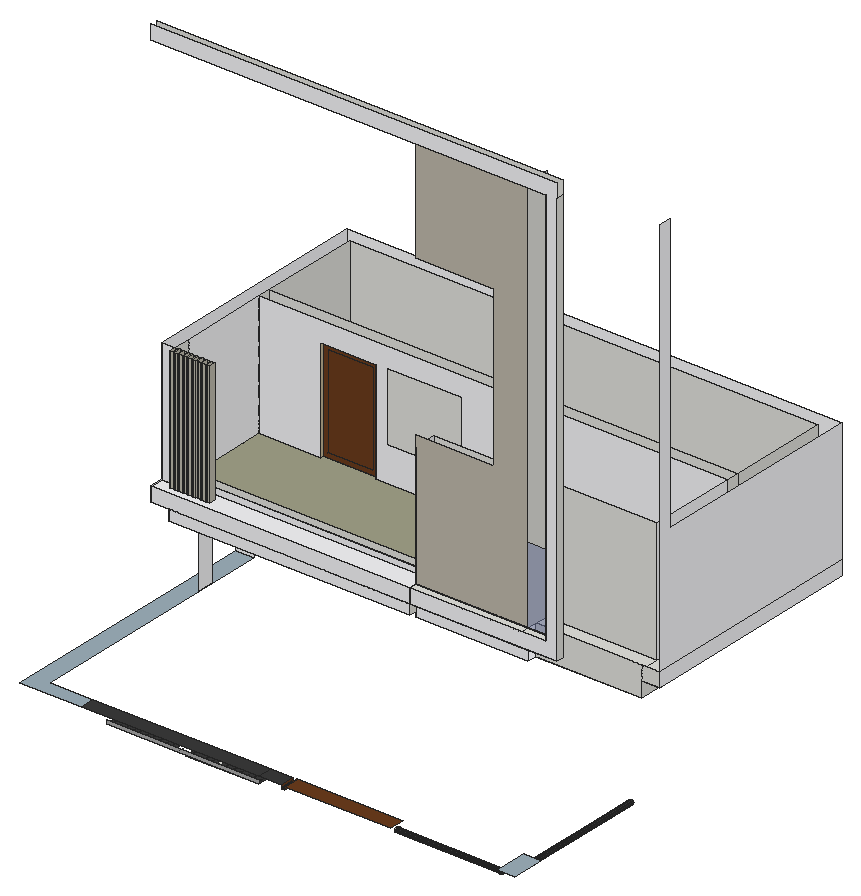
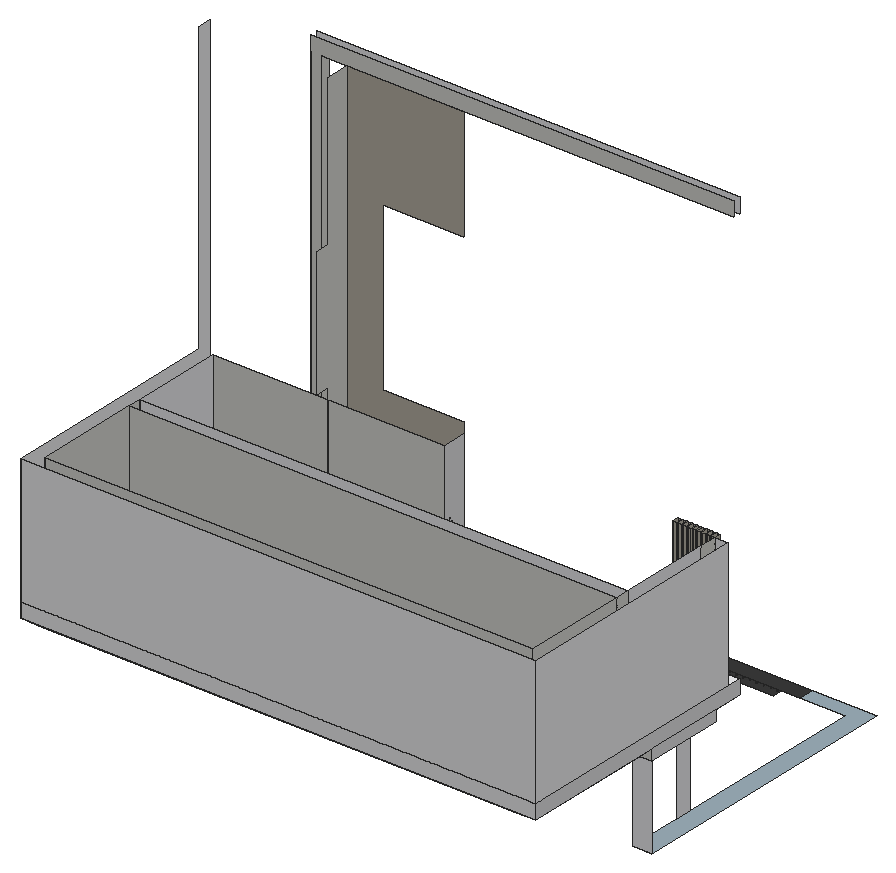
# SketchUp Ruby script. Lengths in inches.
U = 1.inch
M = Sketchup.active_model
def pt(a) = Geom::Point3d.new(a.map { |v| v * U })
def face(e, loops, mat)
  f = e.add_face(loops[0].map { |a| pt(a) })
  loops[1..].each { |l| e.add_face(l.map { |a| pt(a) }).erase! }
  f.material = f.back_material = mat if mat
  f
end
# faces: each face lists its corners as indices into pts; further lists are holes
def faces(e, pts, list, mat = nil) = list.each { |f| face(e, (f[0].is_a?(Array) ? f : [f]).map { |l| l.map { |i| pts[i] } }, mat) }
# xy, xz, yz: faces in a plane at the given z, y or x. An outline is a flat list of corners, or four numbers for a rectangle; further outlines are holes
def ring(l) = l.size == 4 ? [[l[0], l[1]], [l[2], l[1]], [l[2], l[3]], [l[0], l[3]]] : l.each_slice(2).to_a
def flat(e, list, mat, &to3) = list.each { |f| face(e, (f[0].is_a?(Array) ? f : [f]).map { |l| ring(l).map { |u, v| to3.(u, v) } }, mat) }
def xy(e, z, list, mat = nil) = flat(e, list, mat) { |x, y| [x, y, z] }
def xz(e, y, list, mat = nil) = flat(e, list, mat) { |x, z| [x, y, z] }
def yz(e, x, list, mat = nil) = flat(e, list, mat) { |y, z| [x, y, z] }
def lines(e, pts, list) = list.each { |a, b| e.add_line(pt(pts[a]), pt(pts[b])) }
# prism: a flat outline (further loops are holes) pulled along v
def prism(e, loops, v, mat = nil)
  f = face(e, loops, mat); d = Geom::Vector3d.new(v.map { |x| x * U })
  f.pushpull(f.normal.samedirection?(d) ? d.length : -d.length)
end
def box(e, o, s, mat = nil) = prism(e, [[o, [o[0] + s[0], o[1], o[2]], [o[0] + s[0], o[1] + s[1], o[2]], [o[0], o[1] + s[1], o[2]]]], [0, 0, s[2]], mat)
def at(x, y, z, deg = 0) = Geom::Transformation.translation(pt([x, y, z])) * Geom::Transformation.rotation(ORIGIN, Z_AXIS, deg.degrees)
def axes(o, x, y, z) = Geom::Transformation.new([*x, 0, *y, 0, *z, 0, *pt(o).to_a, 1])
def part(name) = M.definitions.add(name)
# library, detail: a bought-in or finely detailed component or shape, given as its bounding box
def library(name, o, s) = part(name).tap { |d| box(d.entities, o, s) }
def detail(e, o, s) = box(e.add_group.entities, o, s)
def put(e, d, t, mat = nil) = e.add_instance(d, t).tap { |i| i.material = mat if mat }
def group(e, t, mat = nil) = e.add_group.tap { |g| g.transformation = t; g.material = mat if mat }.entities
root = M.entities
M.materials.add("[Asphalt New]").color = [67, 60, 62]
M.materials.add("[Blinds Vertical Pattern]").color = [245, 245, 247]
M.materials.add("[Blinds Vertical Pattern]2").color = [234, 234, 237]
M.materials.add("[Blinds Vertical Pattern]3").color = [247, 247, 249]
M.materials.add("[Cinder Block]").color = [191, 184, 171]
M.materials.add("[Color M03]").color = [170, 170, 170]
M.materials.add("[Color M07]").color = [58, 58, 58]
M.materials.add("[Fabric Linen]").color = [161, 161, 136]
M.materials.add("[Formica Beige]").color = [211, 187, 149]
M.materials.add("[Formica Graystone]").color = [191, 187, 173]
M.materials.add("[Formica Speckled Grey]").color = [157, 176, 186]
M.materials.add("[Quartz Light Brown]").color = [199, 184, 152]
M.materials.add("[Quartz Light Grey]").color = [251, 251, 252]
M.materials.add("[Translucent Glass Sky Reflection]").color = [126, 138, 183]
M.materials["[Translucent Glass Sky Reflection]"].alpha = 0.52
M.materials.add("[Wood Cherry Original]").color = [107, 60, 29]
xy(root,112.6,[[[163.91,195.25,260.48,216.53],[167.65,202.87,168.24,202.95,168.8,203.18,169.28,203.55,169.65,204.03,169.88,204.58,169.96,205.18,169.88,205.78,169.65,206.34,169.28,206.82,168.8,207.18,168.24,207.42,167.65,207.49,167.05,207.42,166.49,207.18,166.01,206.82,165.64,206.34,165.41,205.78,165.33,205.18,165.41,204.58,165.64,204.03,166.01,203.55,166.49,203.18,167.05,202.95],[176.58,202.87,177.18,202.95,177.74,203.18,178.22,203.55,178.59,204.03,178.82,204.58,178.9,205.18,178.82,205.78,178.59,206.34,178.22,206.82,177.74,207.18,177.18,207.42,176.58,207.49,175.98,207.42,175.43,207.18,174.95,206.82,174.58,206.34,174.35,205.78,174.27,205.18,174.35,204.58,174.58,204.03,174.95,203.55,175.43,203.18,175.98,202.95],[186.9,202.87,187.49,202.95,188.05,203.18,188.53,203.55,188.9,204.03,189.13,204.58,189.21,205.18,189.13,205.78,188.9,206.34,188.53,206.82,188.05,207.18,187.49,207.42,186.9,207.49,186.3,207.42,185.74,207.18,185.26,206.82,184.89,206.34,184.66,205.78,184.58,205.18,184.66,204.58,184.89,204.03,185.26,203.55,185.74,203.18,186.3,202.95],[196.21,202.87,196.81,202.95,197.36,203.18,197.84,203.55,198.21,204.03,198.44,204.58,198.52,205.18,198.44,205.78,198.21,206.34,197.84,206.82,197.36,207.18,196.81,207.42,196.21,207.49,195.61,207.42,195.05,207.18,194.57,206.82,194.21,206.34,193.97,205.78,193.9,205.18,193.97,204.58,194.21,204.03,194.57,203.55,195.05,203.18,195.61,202.95],[205.65,202.87,206.24,202.95,206.8,203.18,207.28,203.55,207.65,204.03,207.88,204.58,207.96,205.18,207.88,205.78,207.65,206.34,207.28,206.82,206.8,207.18,206.24,207.42,205.65,207.49,205.05,207.42,204.49,207.18,204.01,206.82,203.64,206.34,203.41,205.78,203.33,205.18,203.41,204.58,203.64,204.03,204.01,203.55,204.49,203.18,205.05,202.95],[215.27,202.87,215.87,202.95,216.43,203.18,216.91,203.55,217.27,204.03,217.5,204.58,217.58,205.18,217.5,205.78,217.27,206.34,216.91,206.82,216.43,207.18,215.87,207.42,215.27,207.49,214.67,207.42,214.11,207.18,213.64,206.82,213.27,206.34,213.04,205.78,212.96,205.18,213.04,204.58,213.27,204.03,213.64,203.55,214.11,203.18,214.67,202.95],[224.83,202.87,225.43,202.95,225.99,203.18,226.47,203.55,226.84,204.03,227.07,204.58,227.15,205.18,227.07,205.78,226.84,206.34,226.47,206.82,225.99,207.18,225.43,207.42,224.83,207.49,224.23,207.42,223.68,207.18,223.2,206.82,222.83,206.34,222.6,205.78,222.52,205.18,222.6,204.58,222.83,204.03,223.2,203.55,223.68,203.18,224.23,202.95],[234.71,202.87,235.31,202.95,235.86,203.18,236.34,203.55,236.71,204.03,236.94,204.58,237.02,205.18,236.94,205.78,236.71,206.34,236.34,206.82,235.86,207.18,235.31,207.42,234.71,207.49,234.11,207.42,233.55,207.18,233.07,206.82,232.71,206.34,232.47,205.78,232.4,205.18,232.47,204.58,232.71,204.03,233.07,203.55,233.55,203.18,234.11,202.95],[245.08,202.87,245.68,202.95,246.24,203.18,246.72,203.55,247.09,204.03,247.32,204.58,247.4,205.18,247.32,205.78,247.09,206.34,246.72,206.82,246.24,207.18,245.68,207.42,245.08,207.49,244.48,207.42,243.93,207.18,243.45,206.82,243.08,206.34,242.85,205.78,242.77,205.18,242.85,204.58,243.08,204.03,243.45,203.55,243.93,203.18,244.48,202.95],[254.71,202.87,255.31,202.95,255.86,203.18,256.34,203.55,256.71,204.03,256.94,204.58,257.02,205.18,256.94,205.78,256.71,206.34,256.34,206.82,255.86,207.18,255.31,207.42,254.71,207.49,254.11,207.42,253.55,207.18,253.07,206.82,252.71,206.34,252.47,205.78,252.4,205.18,252.47,204.58,252.71,204.03,253.07,203.55,253.55,203.18,254.11,202.95]],[[280.09,195.25,387.25,216.53],[283.71,202.87,284.31,202.95,284.86,203.18,285.34,203.55,285.71,204.03,285.94,204.58,286.02,205.18,285.94,205.78,285.71,206.34,285.34,206.82,284.86,207.18,284.31,207.42,283.71,207.49,283.11,207.42,282.55,207.18,282.07,206.82,281.71,206.34,281.47,205.78,281.4,205.18,281.47,204.58,281.71,204.03,282.07,203.55,282.55,203.18,283.11,202.95],[292.65,202.87,293.24,202.95,293.8,203.18,294.28,203.55,294.65,204.03,294.88,204.58,294.96,205.18,294.88,205.78,294.65,206.34,294.28,206.82,293.8,207.18,293.24,207.42,292.65,207.49,292.05,207.42,291.49,207.18,291.01,206.82,290.64,206.34,290.41,205.78,290.33,205.18,290.41,204.58,290.64,204.03,291.01,203.55,291.49,203.18,292.05,202.95],[302.65,202.87,303.24,202.95,303.8,203.18,304.28,203.55,304.65,204.03,304.88,204.58,304.96,205.18,304.88,205.78,304.65,206.34,304.28,206.82,303.8,207.18,303.24,207.42,302.65,207.49,302.05,207.42,301.49,207.18,301.01,206.82,300.64,206.34,300.41,205.78,300.33,205.18,300.41,204.58,300.64,204.03,301.01,203.55,301.49,203.18,302.05,202.95],[312.15,202.87,312.74,202.95,313.3,203.18,313.78,203.55,314.15,204.03,314.38,204.58,314.46,205.18,314.38,205.78,314.15,206.34,313.78,206.82,313.3,207.18,312.74,207.42,312.15,207.49,311.55,207.42,310.99,207.18,310.51,206.82,310.14,206.34,309.91,205.78,309.83,205.18,309.91,204.58,310.14,204.03,310.51,203.55,310.99,203.18,311.55,202.95],[332.21,202.87,332.81,202.95,333.36,203.18,333.84,203.55,334.21,204.03,334.44,204.58,334.52,205.18,334.44,205.78,334.21,206.34,333.84,206.82,333.36,207.18,332.81,207.42,332.21,207.49,331.61,207.42,331.05,207.18,330.57,206.82,330.21,206.34,329.97,205.78,329.9,205.18,329.97,204.58,330.21,204.03,330.57,203.55,331.05,203.18,331.61,202.95],[343.15,202.87,343.74,202.95,344.3,203.18,344.78,203.55,345.15,204.03,345.38,204.58,345.46,205.18,345.38,205.78,345.15,206.34,344.78,206.82,344.3,207.18,343.74,207.42,343.15,207.49,342.55,207.42,341.99,207.18,341.51,206.82,341.14,206.34,340.91,205.78,340.83,205.18,340.91,204.58,341.14,204.03,341.51,203.55,341.99,203.18,342.55,202.95],[353.71,202.87,354.31,202.95,354.86,203.18,355.34,203.55,355.71,204.03,355.94,204.58,356.02,205.18,355.94,205.78,355.71,206.34,355.34,206.82,354.86,207.18,354.31,207.42,353.71,207.49,353.11,207.42,352.55,207.18,352.07,206.82,351.71,206.34,351.47,205.78,351.4,205.18,351.47,204.58,351.71,204.03,352.07,203.55,352.55,203.18,353.11,202.95],[363.9,202.87,364.49,202.95,365.05,203.18,365.53,203.55,365.9,204.03,366.13,204.58,366.21,205.18,366.13,205.78,365.9,206.34,365.53,206.82,365.05,207.18,364.49,207.42,363.9,207.49,363.3,207.42,362.74,207.18,362.26,206.82,361.89,206.34,361.66,205.78,361.58,205.18,361.66,204.58,361.89,204.03,362.26,203.55,362.74,203.18,363.3,202.95],[373.96,202.87,374.56,202.95,375.11,203.18,375.59,203.55,375.96,204.03,376.19,204.58,376.27,205.18,376.19,205.78,375.96,206.34,375.59,206.82,375.11,207.18,374.56,207.42,373.96,207.49,373.36,207.42,372.8,207.18,372.32,206.82,371.96,206.34,371.72,205.78,371.65,205.18,371.72,204.58,371.96,204.03,372.32,203.55,372.8,203.18,373.36,202.95],[382.71,202.87,383.31,202.95,383.86,203.18,384.34,203.55,384.71,204.03,384.94,204.58,385.02,205.18,384.94,205.78,384.71,206.34,384.34,206.82,383.86,207.18,383.31,207.42,382.71,207.49,382.11,207.42,381.55,207.18,381.07,206.82,380.71,206.34,380.47,205.78,380.4,205.18,380.47,204.58,380.71,204.03,381.07,203.55,381.55,203.18,382.11,202.95]]],"[Color M07]")
xy(root,113.625,[[322.33,202.87,322.93,202.95,323.49,203.18,323.97,203.55,324.34,204.03,324.57,204.58,324.65,205.18,324.57,205.78,324.34,206.34,323.97,206.82,323.49,207.18,322.93,207.42,322.33,207.49,321.73,207.42,321.18,207.18,320.7,206.82,320.33,206.34,320.1,205.78,320.02,205.18,320.1,204.58,320.33,204.03,320.7,203.55,321.18,203.18,321.73,202.95]])
xy(root,117.97,[[420.08,195.25,425.33,216.53]],"[Asphalt New]")
xy(root,120.22,[[420.08,195.25,425.33,216.53]],"[Asphalt New]")
xy(root,122.8125,[[126.39,195.25,387.25,216.53],[387.25,195.25,420.08,216.53]],"[Color M07]")
xy(root,122.8125,[[36.42,195.25,126.39,195.25,126.39,216.53,62.71,216.53,62.71,590.55,36.42,590.55],[736.96,195.25,761.74,242.62]],"[Formica Speckled Grey]")
xy(root,122.8125,[[425.33,195.25,580.71,216.53]],"[Wood Cherry Original]")
xy(root,213.75,[[168.16,590.55,262.6,602.92]],"[Formica Beige]")
xy(root,231.5625,[[415.32,446.5625,415.32,590.55,735.46,590.55,735.46,461.03,580.71,461.03,580.71,446.5625]],"[Blinds Vertical Pattern]2")
xy(root,238.875,[[[62.71,435.375,62.71,477.68,36.42,477.68,36.42,590.55,399.08,590.55,399.08,461.03,415.32,461.03,415.32,435.375],[62.71,489.78,81.96,513.87]]],"[Blinds Vertical Pattern]2")
xy(root,254.375,[[[62.71,435.375,415.32,435.375,415.32,461.03,399.08,461.03,399.08,590.55,36.42,590.55,36.42,477.68,62.71,477.68],[62.71,489.78,81.96,513.87]],[415.32,435.375,580.71,446.5625],[580.71,435.375,631.7,446.5625],[399.08,461.03,415.32,461.03,415.32,590.55,735.46,590.55,735.46,614.75,399.08,614.75],[735.46,461.03,761.74,590.55],
  [62.71,489.78,81.96,513.87],[36.42,590.55,62.71,614.75],[62.71,590.55,399.08,614.75],[735.46,590.55,761.74,614.75],[36.42,614.75,62.71,794.75],
  [62.71,614.75,735.46,768.47],[735.46,614.75,761.74,794.75],[62.71,768.47,735.46,794.75]])
xy(root,254.375,[[36.42,435.375,62.71,477.68]],"[Blinds Vertical Pattern]2")
xy(root,275.125,[[415.32,435.375,580.71,446.5625],[580.71,435.375,615.19,446.5625],[55.41,446.5625,60.47,455.72],[62.04,446.5625,67.1,455.72],[68.6,446.5625,73.66,455.72],
  [75.22,446.5625,80.29,455.72],[81.79,446.5625,86.85,455.72],[88.47,446.5625,93.54,455.72],[95.47,446.5625,100.54,455.72],[102.35,446.5625,107.41,455.72],
  [109.1,446.5625,114.16,455.72],[415.32,446.5625,580.71,480.02],[36.42,455.72,36.42,794.75,761.74,794.75,761.74,461.03,742.75,461.03,742.75,775.76,55.41,775.76,55.41,455.72],[580.71,461.03,742.75,480.02],[55.41,466.16,415.32,480.02],
  [55.41,609.03,55.41,627.89,742.75,627.89,742.75,609.03,227.47,609.03,227.47,614.22,145.91,614.22,145.91,609.03],[55.41,627.89,742.75,775.76]])
xy(root,275.125,[[[36.42,435.375,415.32,435.375,415.32,466.16,55.41,466.16,55.41,455.72,60.47,455.72,60.47,446.5625,55.41,446.5625,55.41,455.72,36.42,455.72],[75.22,446.5625,80.29,455.72],[95.47,446.5625,100.54,455.72],[68.6,446.5625,73.66,455.72],[62.04,446.5625,67.1,455.72],[88.47,446.5625,93.54,455.72],[109.1,446.5625,114.16,455.72],[102.35,446.5625,107.41,455.72],[81.79,446.5625,86.85,455.72]]],"[Blinds Vertical Pattern]")
xy(root,275.125,[[55.41,480.02,742.75,480.02,742.75,609.03,227.47,609.03,227.47,614.22,145.91,614.22,145.91,609.03,55.41,609.03]],"[Fabric Linen]")
xz(root,195.25,[[420.08,117.97,425.33,120.22]],"[Asphalt New]")
xz(root,195.25,[[163.91,112.6,387.25,118.1875]],"[Color M03]")
xz(root,216.53,[[420.08,117.97,425.33,120.22]],"[Asphalt New]")
xz(root,242.62,[[749.95,112.77,750.79,112.88,751.57,113.2,752.24,113.72,752.76,114.39,753.09,115.18,753.2,116.02,753.09,116.86,752.76,117.64,752.24,118.32,751.57,118.83,750.79,119.16,749.95,119.27,749.11,119.16,748.32,118.83,747.65,118.32,747.13,117.64,746.81,116.86,746.7,116.02,746.81,115.18,747.13,114.39,747.65,113.72,748.32,113.2,749.11,112.88]],"[Quartz Light Grey]")
xz(root,435.375,[[62.71,238.875,415.32,254.375],[36.42,254.375,415.32,275.125],[415.32,254.375,631.7,254.375,631.7,882.375,36.42,882.375,36.42,861.625,615.19,861.625,615.19,275.125,415.32,275.125]],"[Blinds Vertical Pattern]")
xz(root,446.5625,[[415.32,254.375,415.32,275.125,615.19,275.125,615.19,861.625,36.42,861.625,36.42,882.375,631.7,882.375,631.7,254.375]])
xz(root,446.5625,[[415.32,231.5625,580.71,254.375]],"[Blinds Vertical Pattern]")
xz(root,446.5625,[[415.32,275.125,580.71,275.125,580.71,861.625,415.32,861.625,415.32,703.5,530.38,703.5,530.38,470.5625,415.32,470.5625]],"[Cinder Block]")
xz(root,446.5625,[[55.41,275.125,60.47,455.125],[62.04,275.125,67.1,455.125],[68.6,275.125,73.66,455.125],[75.22,275.125,80.29,455.125],[81.79,275.125,86.85,455.125],
  [88.47,275.125,93.54,455.125],[95.47,275.125,100.54,455.125],[102.35,275.125,107.41,455.125],[109.1,275.125,114.16,455.125]],"[Formica Graystone]")
xz(root,446.5625,[[580.71,275.125,615.19,387.88]],"[Translucent Glass Sky Reflection]")
xz(root,455.72,[[36.42,275.125,55.41,455.125]],"[Blinds Vertical Pattern]")
xz(root,455.72,[[55.41,275.125,60.47,455.125],[62.04,275.125,67.1,455.125],[68.6,275.125,73.66,455.125],[75.22,275.125,80.29,455.125],[81.79,275.125,86.85,455.125],
  [88.47,275.125,93.54,455.125],[95.47,275.125,100.54,455.125],[102.35,275.125,107.41,455.125],[109.1,275.125,114.16,455.125]],"[Formica Graystone]")
xz(root,461.03,[[580.71,231.5625,735.46,275.125],[399.08,238.875,415.32,254.375],[735.46,254.375,761.74,275.125]])
xz(root,466.16,[[55.41,275.125,415.32,284.1875]],"[Blinds Vertical Pattern]")
xz(root,477.68,[[36.42,238.875,62.71,254.375]],"[Blinds Vertical Pattern]2")
xz(root,480.02,[[55.41,275.125,415.32,284.1875],[415.32,275.125,580.71,455.125],[580.71,275.125,742.75,455.125]])
xz(root,489.78,[[62.71,238.875,81.96,254.375]])
xz(root,513.87,[[62.71,238.875,81.96,254.375]])
xz(root,590.55,[[415.32,231.5625,735.46,254.375],[36.42,238.875,62.71,254.375],[62.71,238.875,399.08,254.375]])
xz(root,590.55,[[36.42,122.8125,62.71,238.875]],"[Blinds Vertical Pattern]")
xz(root,609.03,[[[55.41,275.125,145.91,275.125,145.91,425.375,227.47,425.375,227.47,275.125,742.75,275.125,742.75,455.125,55.41,455.125],[243.47,326.28,353.18,427.34]]],"[Blinds Vertical Pattern]")
xz(root,614.22,[[[145.91,275.125,227.47,425.375],[152.77,281.99,220.61,418.51]],[152.77,281.99,220.61,418.51]],"[Wood Cherry Original]")
xz(root,627.89,[[55.41,275.125,742.75,455.125]])
xz(root,775.76,[[55.41,275.125,742.75,455.125]])
xz(root,794.75,[[36.42,254.375,761.74,275.125],[36.42,275.125,761.74,455.125]],"[Blinds Vertical Pattern]3")
yz(root,36.42,[[477.68,238.875,590.55,254.375],[435.375,254.375,794.75,275.125]],"[Blinds Vertical Pattern]2")
yz(root,36.42,[[455.72,275.125,794.75,455.125]],"[Blinds Vertical Pattern]3")
yz(root,55.41,[[[455.72,275.125,466.16,275.125,466.16,356.25,480.02,356.25,480.02,455.125,455.72,455.125],[472.17,357.99,471.66,358.05,471.17,358.25,470.76,358.57,470.44,358.99,470.24,359.47,470.17,359.99,470.24,360.5,470.44,360.99,470.76,361.4,471.17,361.72,471.66,361.92,472.17,361.99,472.69,361.92,473.17,361.72,473.59,361.4,473.91,360.99,474.11,360.5,474.17,359.99,474.11,359.47,473.91,358.99,473.59,358.57,473.17,358.25,472.69,358.05]],[466.16,275.125,480.02,284.1875],[609.03,275.125,627.89,455.125],[627.89,275.125,775.76,455.125]])
yz(root,55.41,[[480.02,275.125,609.03,455.125]],"[Blinds Vertical Pattern]")
yz(root,55.41,[[446.5625,275.125,455.72,455.125]],"[Formica Graystone]")
yz(root,60.47,[[446.5625,275.125,455.72,455.125]],"[Formica Graystone]")
yz(root,62.04,[[446.5625,275.125,455.72,455.125]],"[Formica Graystone]")
yz(root,62.71,[[489.78,238.875,513.87,254.375]])
yz(root,62.71,[[489.78,122.8125,513.87,238.875]],"[Blinds Vertical Pattern]")
yz(root,62.71,[[435.375,238.875,477.68,254.375]],"[Blinds Vertical Pattern]2")
yz(root,67.1,[[446.5625,275.125,455.72,455.125]],"[Formica Graystone]")
yz(root,68.6,[[446.5625,275.125,455.72,455.125]],"[Formica Graystone]")
yz(root,73.66,[[446.5625,275.125,455.72,455.125]],"[Formica Graystone]")
yz(root,75.22,[[446.5625,275.125,455.72,455.125]],"[Formica Graystone]")
yz(root,80.29,[[446.5625,275.125,455.72,455.125]],"[Formica Graystone]")
yz(root,81.79,[[446.5625,275.125,455.72,455.125]],"[Formica Graystone]")
yz(root,81.96,[[489.78,238.875,513.87,254.375]])
yz(root,86.85,[[446.5625,275.125,455.72,455.125]],"[Formica Graystone]")
yz(root,88.47,[[446.5625,275.125,455.72,455.125]],"[Formica Graystone]")
yz(root,93.54,[[446.5625,275.125,455.72,455.125]],"[Formica Graystone]")
yz(root,95.47,[[446.5625,275.125,455.72,455.125]],"[Formica Graystone]")
yz(root,100.54,[[446.5625,275.125,455.72,455.125]],"[Formica Graystone]")
yz(root,102.35,[[446.5625,275.125,455.72,455.125]],"[Formica Graystone]")
yz(root,107.41,[[446.5625,275.125,455.72,455.125]],"[Formica Graystone]")
yz(root,109.1,[[446.5625,275.125,455.72,455.125]],"[Formica Graystone]")
yz(root,114.16,[[446.5625,275.125,455.72,455.125]],"[Formica Graystone]")
yz(root,145.91,[[609.03,275.125,614.22,425.375]],"[Quartz Light Brown]")
yz(root,227.47,[[609.03,275.125,614.22,425.375]],"[Quartz Light Brown]")
yz(root,399.08,[[461.03,238.875,590.55,254.375]])
yz(root,415.32,[[446.5625,231.5625,461.03,238.875],[461.03,231.5625,590.55,254.375],[435.375,238.875,446.5625,254.375],[446.5625,238.875,461.03,254.375],[435.375,254.375,446.5625,275.125],
  [466.16,275.125,480.02,284.1875]])
yz(root,415.32,[[[446.5625,275.125,446.5625,455.125,480.02,455.125,480.02,356.25,466.16,356.25,466.16,275.125],[472.17,357.99,472.69,358.05,473.17,358.25,473.59,358.57,473.91,358.99,474.11,359.47,474.17,359.99,474.11,360.5,473.91,360.99,473.59,361.4,473.17,361.72,472.69,361.92,472.17,361.99,471.66,361.92,471.17,361.72,470.76,361.4,470.44,360.99,470.24,360.5,470.17,359.99,470.24,359.47,470.44,358.99,470.76,358.57,471.17,358.25,471.66,358.05]]],"[Blinds Vertical Pattern]2")
yz(root,420.08,[[195.25,117.97,216.53,120.22],[195.25,120.22,216.53,122.8125]],"[Wood Cherry Original]")
yz(root,425.33,[[195.25,117.97,216.53,120.22],[195.25,120.22,216.53,122.8125]],"[Wood Cherry Original]")
yz(root,580.71,[[205.03,113.17,204.24,113.27,203.5,113.58,202.87,114.06,202.38,114.7,202.08,115.4375,201.97,116.23,202.08,117.02,202.38,117.76,202.87,118.4,203.5,118.88,204.24,119.1875,205.03,119.29,205.83,119.1875,206.57,118.88,207.2,118.4,207.6875,117.76,207.99,117.02,208.1,116.23,207.99,115.4375,207.6875,114.7,207.2,114.06,206.57,113.58,205.83,113.27],[446.5625,275.125,446.5625,861.625,480.02,861.625,480.02,650.5625,499.99,650.5625,499.99,470.5625,480.02,470.5625,480.02,275.125]])
yz(root,615.19,[[435.375,275.125,446.5625,861.625]])
yz(root,631.7,[[435.375,254.375,446.5625,861.625]])
yz(root,735.46,[[461.03,231.5625,590.55,254.375]])
yz(root,742.75,[[609.03,275.125,627.89,455.125],[627.89,275.125,775.76,455.125]])
yz(root,742.75,[[480.02,275.125,609.03,455.125]],"[Blinds Vertical Pattern]")
yz(root,761.74,[[461.03,254.375,794.75,275.125],[461.03,275.125,794.75,275.125,794.75,455.125,480.02,455.125,480.02,861.625,461.03,861.625]],"[Blinds Vertical Pattern]3")
p = [[749.95,242.62,112.77],[749.11,242.62,112.88],[749.11,423.625,112.88],[749.95,423.625,112.77],[750.79,242.62,112.88],[750.79,423.625,112.88],
  [748.32,242.62,113.2],[748.32,423.625,113.2],[751.57,242.62,113.2],[751.57,423.625,113.2],[580.71,204.24,113.27],[580.71,205.03,113.17],
  [736.96,205.03,113.17],[736.96,204.24,113.27],[580.71,205.83,113.27],[736.96,205.83,113.27],[747.65,242.62,113.72],[747.65,423.625,113.72],
  [752.24,242.62,113.72],[752.24,423.625,113.72],[580.71,203.5,113.58],[736.96,203.5,113.58],[580.71,206.57,113.58],[736.96,206.57,113.58],
  [580.71,202.87,114.06],[736.96,202.87,114.06],[580.71,207.2,114.06],[736.96,207.2,114.06],[747.13,242.62,114.39],[747.13,423.625,114.39],
  [752.76,242.62,114.39],[752.76,423.625,114.39],[580.71,202.38,114.7],[736.96,202.38,114.7],[580.71,207.6875,114.7],[736.96,207.6875,114.7],
  [746.81,242.62,115.18],[746.81,423.625,115.18],[753.09,242.62,115.18],[753.09,423.625,115.18],[580.71,202.08,115.4375],[736.96,202.08,115.4375],
  [580.71,207.99,115.4375],[736.96,207.99,115.4375],[746.7,242.62,116.02],[746.7,423.625,116.02],[753.2,242.62,116.02],[753.2,423.625,116.02],
  [580.71,201.97,116.23],[736.96,201.97,116.23],[580.71,208.1,116.23],[736.96,208.1,116.23],[746.81,242.62,116.86],[746.81,423.625,116.86],
  [753.09,242.62,116.86],[753.09,423.625,116.86],[580.71,202.08,117.02],[736.96,202.08,117.02],[580.71,207.99,117.02],[736.96,207.99,117.02],
  [747.13,242.62,117.64],[747.13,423.625,117.64],[752.76,242.62,117.64],[752.76,423.625,117.64],[580.71,202.38,117.76],[736.96,202.38,117.76],
  [580.71,207.6875,117.76],[736.96,207.6875,117.76],[747.65,242.62,118.32],[747.65,423.625,118.32],[752.24,242.62,118.32],[752.24,423.625,118.32],
  [580.71,202.87,118.4],[736.96,202.87,118.4],[580.71,207.2,118.4],[736.96,207.2,118.4],[748.32,242.62,118.83],[748.32,423.625,118.83],
  [751.57,242.62,118.83],[751.57,423.625,118.83],[580.71,203.5,118.88],[736.96,203.5,118.88],[580.71,206.57,118.88],[736.96,206.57,118.88],
  [749.11,242.62,119.16],[749.11,423.625,119.16],[750.79,242.62,119.16],[750.79,423.625,119.16],[580.71,204.24,119.1875],[736.96,204.24,119.1875],
  [580.71,205.83,119.1875],[736.96,205.83,119.1875],[580.71,205.03,119.29],[736.96,205.03,119.29],[749.95,242.62,119.27],[749.95,423.625,119.27],
  [270.29,216.53,115.66],[270.29,195.25,115.66]]
faces(root,p,[[0,1,2,3],[4,0,3,5],[1,6,7,2],[8,4,5,9],[10,11,12,13],[11,14,15,12],[6,16,17,7],[18,8,9,19],
  [20,10,13,21],[14,22,23,15],[24,20,21,25],[22,26,27,23],[16,28,29,17],[30,18,19,31],[32,24,25,33],[26,34,35,27],
  [28,36,37,29],[38,30,31,39],[40,32,33,41],[34,42,43,35],[36,44,45,37],[46,38,39,47],[48,40,41,49],[42,50,51,43],
  [44,52,53,45],[54,46,47,55],[56,48,49,57],[50,58,59,51],[52,60,61,53],[62,54,55,63],[64,56,57,65],[58,66,67,59],
  [60,68,69,61],[70,62,63,71],[72,64,65,73],[66,74,75,67],[68,76,77,69],[78,70,71,79],[80,72,73,81],[74,82,83,75],
  [76,84,85,77],[86,78,79,87],[88,80,81,89],[82,90,91,83],[92,88,89,93],[90,92,93,91],[84,94,95,85],[94,86,87,95]],"[Color M07]")
lines(root,p,[[96,97]])
